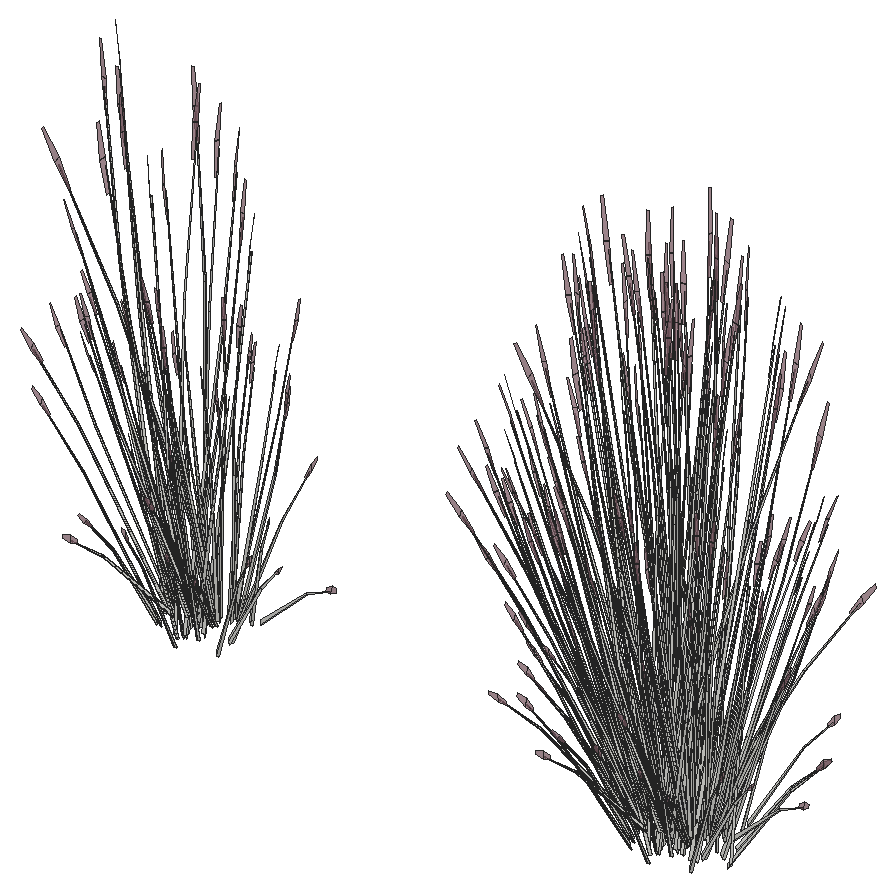
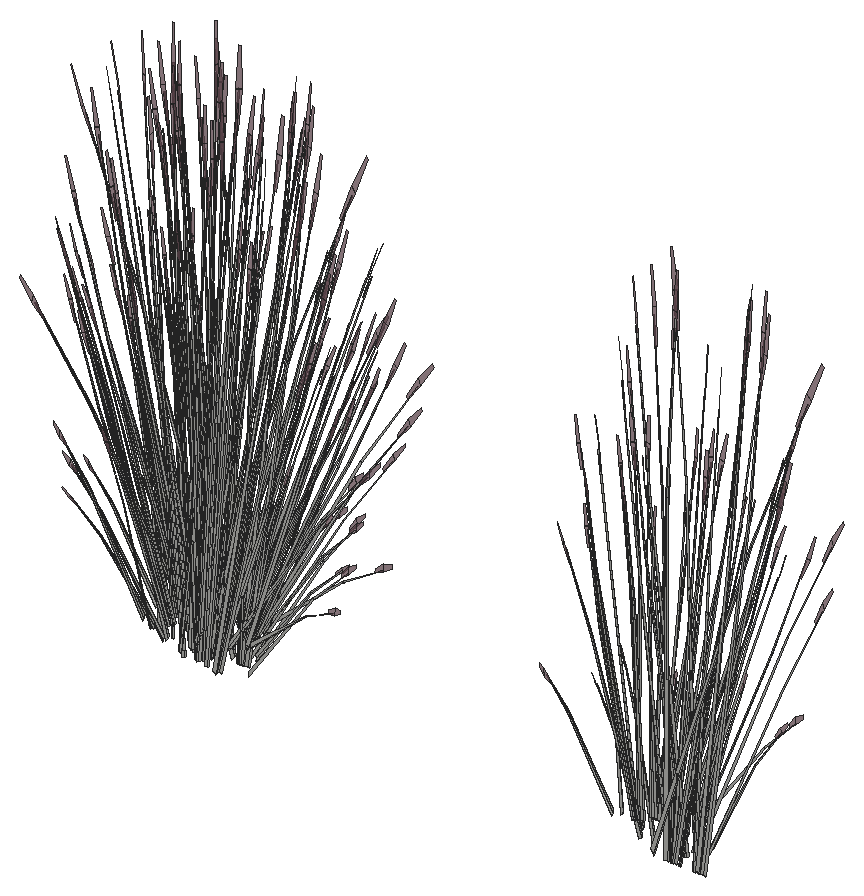
# SketchUp Ruby script. Lengths in inches.
U = 1.inch
M = Sketchup.active_model
def pt(a) = Geom::Point3d.new(a.map { |v| v * U })
def face(e, loops, mat)
  f = e.add_face(loops[0].map { |a| pt(a) })
  loops[1..].each { |l| e.add_face(l.map { |a| pt(a) }).erase! }
  f.material = f.back_material = mat if mat
  f
end
# faces: each face lists its corners as indices into pts; further lists are holes
def faces(e, pts, list, mat = nil) = list.each { |f| face(e, (f[0].is_a?(Array) ? f : [f]).map { |l| l.map { |i| pts[i] } }, mat) }
# xy, xz, yz: faces in a plane at the given z, y or x. An outline is a flat list of corners, or four numbers for a rectangle; further outlines are holes
def ring(l) = l.size == 4 ? [[l[0], l[1]], [l[2], l[1]], [l[2], l[3]], [l[0], l[3]]] : l.each_slice(2).to_a
def flat(e, list, mat, &to3) = list.each { |f| face(e, (f[0].is_a?(Array) ? f : [f]).map { |l| ring(l).map { |u, v| to3.(u, v) } }, mat) }
def xy(e, z, list, mat = nil) = flat(e, list, mat) { |x, y| [x, y, z] }
def xz(e, y, list, mat = nil) = flat(e, list, mat) { |x, z| [x, y, z] }
def yz(e, x, list, mat = nil) = flat(e, list, mat) { |y, z| [x, y, z] }
def lines(e, pts, list) = list.each { |a, b| e.add_line(pt(pts[a]), pt(pts[b])) }
# prism: a flat outline (further loops are holes) pulled along v
def prism(e, loops, v, mat = nil)
  f = face(e, loops, mat); d = Geom::Vector3d.new(v.map { |x| x * U })
  f.pushpull(f.normal.samedirection?(d) ? d.length : -d.length)
end
def box(e, o, s, mat = nil) = prism(e, [[o, [o[0] + s[0], o[1], o[2]], [o[0] + s[0], o[1] + s[1], o[2]], [o[0], o[1] + s[1], o[2]]]], [0, 0, s[2]], mat)
def at(x, y, z, deg = 0) = Geom::Transformation.translation(pt([x, y, z])) * Geom::Transformation.rotation(ORIGIN, Z_AXIS, deg.degrees)
def axes(o, x, y, z) = Geom::Transformation.new([*x, 0, *y, 0, *z, 0, *pt(o).to_a, 1])
def part(name) = M.definitions.add(name)
# library, detail: a bought-in or finely detailed component or shape, given as its bounding box
def library(name, o, s) = part(name).tap { |d| box(d.entities, o, s) }
def detail(e, o, s) = box(e.add_group.entities, o, s)
def put(e, d, t, mat = nil) = e.add_instance(d, t).tap { |i| i.material = mat if mat }
def group(e, t, mat = nil) = e.add_group.tap { |g| g.transformation = t; g.material = mat if mat }.entities
root = M.entities
M.materials.add("LightPink_Translucent").color = [144, 107, 117]
M.materials["LightPink_Translucent"].alpha = 0.75
c1 = part("blade")
p = [[2.15,0.21,22],[0,0.17,0],[0.09,0.45,0],[2.18,0.31,22],[2.29,0.31,22],[0.38,0.45,0],
  [2.48,0.24,33],[2.49,0.24,33],[2.48,0.22,33]]
faces(c1.entities,p,[[0,1,2,3],[4,5,2,3],[6,3,4,7],[8,0,3,6]])
c2 = part("seeds")
p = [[0.3,-0.1,1.38],[-0.01,-0.03,1.59],[-0.01,-0.03,0.03],[0.14,-0.07,-0.07],[0.29,-0.03,3],[0.15,0.01,3.11]]
faces(c2.entities,p,[[0,1,2,3],[1,0,4,5]],"LightPink_Translucent")
c3 = part("blade with seeds")
put(c3.entities,c1,at(0,0,0))
put(c3.entities,c2,axes([2.4,0.25,30.99],[1.5799,-0.05474,1.17369],[-0.12525,1.92788,0.29478],[-0.07173,-0.02425,1.56792]))
put(root,c3,axes([752.32,276.33,1.9375],[0.10505,0.10498,0.85688],[-0.48542,0.08838,0.06928],[-0.10971,-0.1648,0.36631]))
put(root,c3,axes([753.12,275.64,2.36],[-0.07029,-0.04584,0.87472],[-0.46908,0.02906,-0.13834],[-0.07486,-0.10965,0.07015]))
put(root,c3,axes([754.21,276.18,1.3],[-0.13063,0.06618,0.71501],[-0.39122,-0.11583,-0.15377],[0.07252,-0.14406,0.3057]))
put(root,c3,axes([753.61,276.41,2.49],[-0.21934,-0.26585,-0.35523],[0.45151,-0.14816,0.04287],[-0.05129,-0.12845,0.5025]))
put(root,c3,axes([752.18,276.05,1.3],[-0.02783,0.10696,0.71501],[-0.40683,0.08954,-0.15377],[-0.0951,-0.13825,0.3057]))
put(root,c3,axes([753.23,275.82,0.75],[-0.07708,0.01178,0.88171],[-0.42627,-0.1326,-0.1347],[0.00715,-0.1106,0.15018]))
put(root,c3,axes([754.52,276.67,2.49],[0.01196,-0.30243,-0.35523],[0.50354,0.02031,0.04287],[0.05314,-0.12813,0.5025]))
put(root,c3,axes([755.23,276.2,2.36],[-0.00444,-0.06507,0.87472],[-0.37468,-0.18807,-0.13834],[0.05793,-0.114,0.07015]))
put(root,c3,axes([753.65,276.18,2.26],[0.13855,-0.25143,-0.17707],[0.4042,0.07334,0.2286],[-0.03706,-0.10123,0.4374]))
put(root,c3,axes([753.96,276.52,1.9375],[-0.08557,0.11238,0.85688],[-0.35897,-0.23257,0.06928],[0.16194,-0.14495,0.36631]))
put(root,c3,axes([755.125,275.96,2.35],[-0.04667,0.02497,0.88692],[-0.45726,-0.08426,-0.08381],[-0.01655,-0.10898,0.15695]))
put(root,c3,axes([753.45,276.36,2.34],[-0.45175,-0.08196,-0.25549],[0.15485,-0.28101,-0.1979],[-0.04142,-0.11314,0.48886]))
put(root,c3,axes([753.73,275.65,1.38],[0.05895,0.19066,0.5743],[-0.32704,-0.1056,0.42196],[0.03519,-0.09762,0.12649]))
put(root,c3,axes([754.42,276.57,2.34],[-0.32898,-0.21969,-0.25549],[0.34753,-0.1924,-0.1979],[0.05006,-0.11162,0.48886]))
put(root,c3,axes([752.64,275.49,2.35],[-0.00857,0.03919,0.88692],[-0.42284,0.14223,-0.08381],[-0.12443,-0.0727,0.15695]))
put(root,c3,axes([752.54,276.18,2.55],[0.51193,-0.08404,0.26881],[0.08885,0.32966,0.22165],[-0.1204,-0.09716,0.55625]))
put(root,c3,axes([753.7,276.24,2.37],[0.45283,0.08548,0.24001],[-0.15485,0.28101,0.1979],[-0.02721,-0.11051,0.49665]))
put(root,c3,axes([753.83,276.34,2.52],[-0.44971,0.15222,-0.0608],[-0.221,-0.27017,-0.33747],[-0.05933,-0.11385,0.51278]))
put(root,c3,axes([754.77,276.6875,2.52],[-0.50507,-0.0162,-0.0608],[0.01381,-0.30672,-0.33747],[0.03508,-0.11813,0.51278]))
put(root,c3,axes([754.73,276.49,2.26],[0.31095,-0.17214,-0.17707],[0.29435,0.19656,0.2286],[0.04479,-0.09987,0.4374]))
put(root,c3,axes([752.04,275.88,1.38],[0.23972,0.1138,0.5743],[-0.34912,0.06841,0.42196],[-0.0747,-0.08746,0.12649]))
put(root,c3,axes([753.82,276.22,2.37],[0.33863,-0.11112,0.03215],[0.16575,0.20263,0.2531],[-0.0327,-0.08932,0.38595]))
put(root,c3,axes([752.62,276.49,2.49],[-0.39186,-0.15803,-0.35523],[0.27849,-0.27693,0.04287],[-0.14198,-0.09436,0.5025]))
put(root,c3,axes([752.49,276.28,2.26],[-0.07098,-0.26335,-0.17707],[0.40574,-0.06954,0.2286],[-0.10898,-0.07547,0.4374]))
put(root,c3,axes([752.66,276.25,2.37],[0.20887,-0.2077,0.03215],[0.29744,0.12092,0.2531],[-0.09616,-0.06659,0.38595]))
put(root,c3,axes([751.85,276.23,0.75],[-0.04451,0.04307,0.88171],[-0.44986,0.09286,-0.1347],[-0.10868,-0.08448,0.15018]))
put(root,c3,axes([752.6,277.41,1.05],[-0.18873,-0.33528,-0.34918],[0.54365,-0.12075,-0.09164],[-0.02086,-0.11353,0.77075]))
put(root,c3,axes([751.61,276.66,1.9375],[0.1707,0.05633,0.85688],[-0.35326,0.23632,0.06928],[-0.22018,-0.10661,0.36631]))
put(root,c3,axes([755.12,276.38,0.75],[-0.06878,-0.02576,0.88171],[-0.17668,-0.28776,-0.1347],[0.11919,-0.07809,0.15018]))
put(root,c3,axes([753.7,276.45,2.53],[-0.13855,0.25143,0.17707],[-0.4042,-0.07334,-0.2286],[-0.03706,-0.10123,0.4374]))
put(root,c3,axes([752.4375,276.49,2.34],[-0.45348,0.07772,-0.25549],[-0.07933,-0.29434,-0.1979],[-0.1218,-0.08435,0.48886]))
put(root,c3,axes([754.73,276.56,2.37],[0.32725,0.22308,0.24001],[-0.34753,0.1924,0.1979],[0.06036,-0.10466,0.49665]))
put(root,c3,axes([752.76,276.23,2.72],[-0.30671,0.31344,-0.0681],[-0.44417,-0.18058,-0.37797],[-0.1544,-0.08856,0.57432]))
put(root,c3,axes([754.85,276.58,2.37],[0.37765,0.01523,0.03215],[-0.01035,0.23004,0.2531],[0.03952,-0.08812,0.38595]))
put(root,c3,axes([754.57,276.73,2.53],[-0.31095,0.17214,0.17707],[-0.29435,-0.19656,-0.2286],[0.04479,-0.09987,0.4374]))
put(root,c3,axes([755.12,277.2,2.49],[0.24005,-0.25798,-0.35523],[0.42065,0.18334,0.04287],[0.14333,-0.09347,0.5025]))
put(root,c3,axes([752.52,276.45,1.1875],[-0.28732,-0.32763,0],[0.4807,-0.18271,-0.25804],[0.10948,-0.04161,0.81856]))
put(root,c3,axes([755.11,277.08,2.34],[-0.11806,-0.29854,-0.25549],[0.44709,-0.05222,-0.1979],[0.12812,-0.08019,0.48886]))
put(root,c3,axes([753.15,276.05,1.0625],[-0.31757,0.18757,-0.01946],[-0.29098,-0.20543,-0.08825],[-0.02049,-0.05821,0.29107]))
put(root,c3,axes([751.58,276.14,2.36],[-0.09888,-0.00231,0.87472],[-0.3148,0.23079,-0.13834],[-0.16797,-0.04716,0.07015]))
put(root,c3,axes([755.32,277.29,2.52],[-0.4251,-0.18028,-0.0608],[0.24491,-0.26108,-0.33747],[0.1201,-0.09075,0.51278]))
put(root,c3,axes([753.56,278.27,1.66],[0.39713,0.13184,0.7563],[-0.38905,0.28403,0.29908],[-0.17427,-0.16834,0.63403]))
put(root,c3,axes([752.73,276.49,2.53],[0.07098,0.26335,0.17707],[-0.40574,0.06954,-0.2286],[-0.10898,-0.07547,0.4374]))
put(root,c3,axes([751.48,277.36,1.01],[0,-0.32696,-0.24825],[0.51416,0,0],[0,-0.07447,0.78752]))
put(root,c3,axes([752.91,276.39,1.01],[0.4301,-0.16348,-0.24825],[0.25708,0.29314,0],[0.09796,-0.03723,0.78752]))
put(root,c3,axes([755.46,276.96,1.3],[-0.16417,-0.00968,0.71501],[-0.16819,-0.25979,-0.15377],[0.20169,-0.07349,0.3057]))
put(root,c3,axes([751.51,276.66,2.55],[0.37952,-0.24129,0.26881],[0.32731,0.25625,0.22165],[-0.17806,-0.04451,0.55625]))
put(root,c3,axes([756.36,277.21,2.35],[-0.06002,-0.00248,0.88692],[-0.24926,-0.26607,-0.08381],[0.1001,-0.08748,0.15695]))
put(root,c3,axes([724.19,278.45,1.9375],[0.10505,0.10498,0.85688],[-0.48542,0.08838,0.06928],[-0.10971,-0.1648,0.36631]))
put(root,c3,axes([753.42,277.06,1.03],[0.30954,-0.24575,-0.31177],[0.38452,0.22284,-0.08182],[0.12404,-0.0613,0.68817]))
put(root,c3,axes([755.65,276.48,1.38],[-0.15307,0.16644,0.5743],[-0.13157,-0.22361,0.42196],[0.12643,-0.05603,0.12649]))
put(root,c3,axes([725,277.75,2.36],[-0.07029,-0.04584,0.87472],[-0.46908,0.02906,-0.13834],[-0.07486,-0.10965,0.07015]))
put(root,c3,axes([726.08,278.3,1.3],[-0.13063,0.06618,0.71501],[-0.39122,-0.11583,-0.15377],[0.07252,-0.14406,0.3057]))
put(root,c3,axes([725.49,278.53,2.49],[-0.21934,-0.26585,-0.35523],[0.45151,-0.14816,0.04287],[-0.05129,-0.12845,0.5025]))
put(root,c3,axes([755.43,277.11,2.26],[0.40003,-0.04673,-0.17707],[0.10563,0.26712,0.2286],[0.11464,-0.07175,0.4374]))
put(root,c3,axes([751.68,276.66,2.37],[0.02314,-0.24862,0.03215],[0.34943,0.00682,0.2531],[-0.13385,-0.02602,0.38595]))
put(root,c3,axes([724.0625,278.17,1.3],[-0.02783,0.10696,0.71501],[-0.40683,0.08954,-0.15377],[-0.0951,-0.13825,0.3057]))
put(root,c3,axes([752.88,277.5,1.11],[0.22297,-0.29461,-0.2237],[0.4633,0.14179,0.10766],[0,-0.06791,0.71822]))
put(root,c3,axes([751.55,276.74,2.26],[-0.26148,-0.20471,-0.17707],[0.29857,-0.19378,0.2286],[-0.1517,-0.02948,0.4374]))
put(root,c3,axes([753.09,277.35,1.33],[-0.05355,-0.37308,-0.14548],[0.55775,-0.02256,-0.25001],[0.09822,-0.04969,0.79854]))
put(root,c3,axes([725.11,277.9375,0.75],[-0.07708,0.01178,0.88171],[-0.42627,-0.1326,-0.1347],[0.00715,-0.1106,0.15018]))
put(root,c3,axes([751.7,277.37,1.01],[0.32079,-0.20399,-0.15489],[0.32079,0.20399,0.15489],[0,-0.06571,0.69487]))
put(root,c3,axes([751.57,276.39,1.0625],[-0.13257,0.26698,-0.01946],[-0.40802,-0.08212,-0.08825],[-0.06195,-0.04367,0.29107]))
put(root,c3,axes([755.11,277.26,2.53],[-0.40003,0.04673,0.17707],[-0.10563,-0.26712,-0.2286],[0.11464,-0.07175,0.4374]))
put(root,c3,axes([752.83,277.74,1.33],[-0.51755,-0.15601,-0.14548],[0.2492,-0.32927,-0.25001],[-0.01626,-0.08084,0.79854]))
put(root,c3,axes([751.36,277.61,1.1875],[-0.57465,0,0],[0,-0.36542,-0.25804],[0,-0.08323,0.81856]))
put(root,c3,axes([726.4,278.79,2.49],[0.01196,-0.30243,-0.35523],[0.50354,0.02031,0.04287],[0.05314,-0.12813,0.5025]))
put(root,c3,axes([751.45,276.96,1.3],[0.08973,0.09103,0.71501],[-0.20675,0.24743,-0.15377],[-0.2123,-0.05914,0.3057]))
put(root,c3,axes([753.01,276.52,1.01],[0.42874,0.0809,-0.15489],[-0.10795,0.28489,0.15489],[0.08643,-0.03285,0.69487]))
put(root,c3,axes([727.1,278.31,2.36],[-0.00444,-0.06507,0.87472],[-0.37468,-0.18807,-0.13834],[0.05793,-0.114,0.07015]))
put(root,c3,axes([725.53,278.3,2.26],[0.13855,-0.25143,-0.17707],[0.4042,0.07334,0.2286],[-0.03706,-0.10123,0.4374]))
put(root,c3,axes([725.83,278.63,1.9375],[-0.08557,0.11238,0.85688],[-0.35897,-0.23257,0.06928],[0.16194,-0.14495,0.36631]))
put(root,c3,axes([727,278.08,2.35],[-0.04667,0.02497,0.88692],[-0.45726,-0.08426,-0.08381],[-0.01655,-0.10898,0.15695]))
put(root,c3,axes([751.82,276.875,2.49],[-0.45939,-0.00787,-0.35523],[0.03085,-0.3315,0.04287],[-0.19462,-0.03498,0.5025]))
put(root,c3,axes([725.32,278.47,2.34],[-0.45175,-0.08196,-0.25549],[0.15485,-0.28101,-0.1979],[-0.04142,-0.11314,0.48886]))
put(root,c3,axes([725.6,277.77,1.38],[0.05895,0.19066,0.5743],[-0.32704,-0.1056,0.42196],[0.03519,-0.09762,0.12649]))
put(root,c3,axes([726.3,278.6875,2.34],[-0.32898,-0.21969,-0.25549],[0.34753,-0.1924,-0.1979],[0.05006,-0.11162,0.48886]))
put(root,c3,axes([755.47,277.22,2.37],[0.31549,0.13751,0.03215],[-0.18368,0.19581,0.2531],[0.10115,-0.06331,0.38595]))
put(root,c3,axes([755.38,277.16,2.37],[0.11397,0.30091,0.24001],[-0.44709,0.05222,0.1979],[0.13177,-0.07077,0.49665]))
put(root,c3,axes([756.59,277.53,2.36],[0.06377,-0.0498,0.87472],[-0.08162,-0.30549,-0.13834],[0.16001,-0.05792,0.07015]))
put(root,c3,axes([751.8,277.51,1.17],[-0.42746,0.27488,0.15378],[-0.42772,-0.27199,-0.18246],[-0.01493,-0.07806,0.82443]))
put(root,c3,axes([751.2,276.34,2.35],[0.03407,0.03263,0.88692],[-0.16424,0.29331,-0.08381],[-0.16634,0.00212,0.15695]))
put(root,c3,axes([724.42,278.3,2.55],[0.51193,-0.08404,0.26881],[0.08885,0.32966,0.22165],[-0.1204,-0.09716,0.55625]))
put(root,c3,axes([725.58,278.36,2.37],[0.45283,0.08548,0.24001],[-0.15485,0.28101,0.1979],[-0.02721,-0.11051,0.49665]))
put(root,c3,axes([725.71,278.46,2.52],[-0.44971,0.15222,-0.0608],[-0.221,-0.27017,-0.33747],[-0.05933,-0.11385,0.51278]))
put(root,c3,axes([753.16,277.64,1.22],[0.5178,0.15847,0.12032],[-0.2492,0.32927,0.25001],[0,-0.0759,0.80271]))
put(root,c3,axes([752.96,278.09,1.22],[0.1218,-0.38743,-0.11714],[0.57753,0.06753,0.25635],[-0.10091,-0.0535,0.7822]))
put(root,c3,axes([726.64,278.8,2.52],[-0.50507,-0.0162,-0.0608],[0.01381,-0.30672,-0.33747],[0.03508,-0.11813,0.51278]))
put(root,c3,axes([726.61,278.61,2.26],[0.31095,-0.17214,-0.17707],[0.29435,0.19656,0.2286],[0.04479,-0.09987,0.4374]))
put(root,c3,axes([723.92,278,1.38],[0.23972,0.1138,0.5743],[-0.34912,0.06841,0.42196],[-0.0747,-0.08746,0.12649]))
put(root,c3,axes([725.7,278.34,2.37],[0.33863,-0.11112,0.03215],[0.16575,0.20263,0.2531],[-0.0327,-0.08932,0.38595]))
put(root,c3,axes([751.67,276.94,2.34],[-0.3337,0.21658,-0.25549],[-0.29224,-0.22879,-0.1979],[-0.16955,-0.03295,0.48886]))
put(root,c3,axes([724.36,278.39,2.26],[-0.07098,-0.26335,-0.17707],[0.40574,-0.06954,0.2286],[-0.10898,-0.07547,0.4374]))
put(root,c3,axes([751.92,276.85,2.53],[0.26148,0.20471,0.17707],[-0.29857,0.19378,-0.2286],[-0.1517,-0.02948,0.4374]))
put(root,c3,axes([750.92,277.23,1.38],[0.2934,-0.0234,0.5743],[-0.18611,0.20614,0.42196],[-0.14499,-0.03092,0.12649]))
put(root,c3,axes([752.99,277.42,1.36],[-0.49904,0.02018,0.2237],[-0.04513,-0.33504,-0.10766],[0.08934,-0.03396,0.71822]))
put(root,c3,axes([751.85,276.72,2.52],[-0.02461,0.33251,-0.0608],[-0.4659,-0.00909,-0.33747],[-0.17944,-0.0231,0.51278]))
put(root,c3,axes([751.7,277.67,1.24],[0,0.32696,0.24825],[-0.51416,0,0],[0,-0.07447,0.78752]))
put(root,c3,axes([755.33,277.99,2.52],[-0.23123,-0.29606,-0.0608],[0.41039,-0.14549,-0.33747],[0.17294,-0.03906,0.51278]))
put(root,c3,axes([755.3125,277.74,2.34],[0.1245,-0.29741,-0.25549],[0.42685,0.10194,-0.1979],[0.17186,-0.02727,0.48886]))
put(root,c3,axes([754.64,276.53,1.1875],[0.28732,-0.32763,0],[0.4807,0.18271,-0.25804],[0.10948,0.04161,0.81856]))
put(root,c3,axes([751.25,277.17,1.9375],[0.19062,-0.00741,0.85688],[-0.12645,0.32094,0.06928],[-0.27165,-0.01985,0.36631]))
put(root,c3,axes([752.92,277.93,1.11],[-0.27607,-0.27443,-0.2237],[0.41817,-0.19325,0.10766],[-0.08934,-0.03396,0.71822]))
put(root,c3,axes([752.97,277.54,1.18],[0.1998,0.3656,0.22877],[-0.5709,0.12713,0.08977],[0.00698,-0.06718,0.79428]))
put(root,c3,axes([724.54,278.37,2.37],[0.20887,-0.2077,0.03215],[0.29744,0.12092,0.2531],[-0.09616,-0.06659,0.38595]))
put(root,c3,axes([755.77,277.82,0.99],[-0.29599,0.03924,0.70792],[-0.04711,-0.31232,0.04052],[0.20731,-0.04727,0.40283]))
put(root,c3,axes([756.31,277.55,1.13],[-0.28491,-0.20907,-0.03244],[0.31204,-0.19157,-0.14708],[0.08842,-0.01349,0.48512]))
put(root,c3,axes([724.47,279.53,1.05],[-0.18873,-0.33528,-0.34918],[0.54365,-0.12075,-0.09164],[-0.02086,-0.11353,0.77075]))
put(root,c3,axes([727,278.5,0.75],[-0.06878,-0.02576,0.88171],[-0.17668,-0.28776,-0.1347],[0.11919,-0.07809,0.15018]))
put(root,c3,axes([752.875,277.83,1.36],[-0.22297,0.29461,0.2237],[-0.4633,-0.14179,-0.10766],[0,-0.06791,0.71822]))
put(root,c3,axes([753.69,277.57,1.1],[0,-0.37831,0],[0.57465,0,0],[0,0,0.89728]))
put(root,c3,axes([754.39,276.7,1.24],[-0.4301,-0.16348,0.24825],[0.25708,-0.29314,0],[0.09796,0.03723,0.78752]))
put(root,c3,axes([725.57,278.57,2.53],[-0.13855,0.25143,0.17707],[-0.4042,-0.07334,-0.2286],[-0.03706,-0.10123,0.4374]))
put(root,c3,axes([755.23,277.85,2.49],[0.40382,-0.1444,-0.35523],[0.22505,0.29724,0.04287],[0.19512,-0.03377,0.5025]))
put(root,c3,axes([726.61,278.67,2.37],[0.32725,0.22308,0.24001],[-0.34753,0.1924,0.1979],[0.06036,-0.10466,0.49665]))
put(root,c3,axes([752.67,278.03,1.03],[-0.47805,-0.0536,-0.31177],[0.10088,-0.33065,-0.08182],[-0.14266,-0.04007,0.68817]))
put(root,c3,axes([726.73,278.69,2.37],[0.37765,0.01523,0.03215],[-0.01035,0.23004,0.2531],[0.03952,-0.08812,0.38595]))
put(root,c3,axes([753.42,277.33,1.18],[-0.38104,0.29672,0.22877],[-0.45269,-0.26192,0.08977],[0.09186,-0.02961,0.79428]))
put(root,c3,axes([753.84,277.87,1.15],[-0.42746,-0.28142,-0.03066],[0.42772,-0.28159,0],[-0.01493,-0.00983,0.87786]))
put(root,c3,axes([726.45,278.85,2.53],[-0.31095,0.17214,0.17707],[-0.29435,-0.19656,-0.2286],[0.04479,-0.09987,0.4374]))
put(root,c3,axes([752.76,276.85,1.24],[-0.13276,0.32494,0.08821],[-0.4858,-0.09195,0.17543],[0.08392,-0.00158,0.80203]))
put(root,c3,axes([755.17,277.9,2.53],[-0.38192,-0.09121,0.17707],[0.11139,-0.2661,-0.2286],[0.15377,-0.0244,0.4374]))
put(root,c3,axes([726.99,279.3125,2.49],[0.24005,-0.25798,-0.35523],[0.42065,0.18334,0.04287],[0.14333,-0.09347,0.5025]))
put(root,c3,axes([724.4,278.5625,1.1875],[-0.28732,-0.32763,0],[0.4807,-0.18271,-0.25804],[0.10948,-0.04161,0.81856]))
put(root,c3,axes([726.98,279.19,2.34],[-0.11806,-0.29854,-0.25549],[0.44709,-0.05222,-0.1979],[0.12812,-0.08019,0.48886]))
put(root,c3,axes([751.17,277.42,2.37],[0.12984,-0.29812,0.24001],[0.42685,0.10194,0.1979],[-0.16786,0.01792,0.49665]))
put(root,c3,axes([752.56,277.11,0.8],[-0.45234,0.1309,0.64464],[-0.14398,-0.37559,0.25048],[0.27777,0.00625,0.73321]))
put(root,c3,axes([753.77,277.21,1.31],[0.08866,-0.29179,0.0724],[0.43315,0.05065,-0.20674],[0.07883,0.02996,0.63372]))
put(root,c3,axes([725.03,278.17,1.0625],[-0.31757,0.18757,-0.01946],[-0.29098,-0.20543,-0.08825],[-0.02049,-0.05821,0.29107]))
put(root,c3,axes([751.14,277.34,2.37],[-0.16879,-0.22293,0.03215],[0.30779,-0.10912,0.2531],[-0.13568,0.02153,0.38595]))
put(root,c3,axes([753.02,277.9,1.18],[0.58084,0.06889,0.22877],[-0.11821,0.38906,0.08977],[-0.08488,-0.03757,0.79428]))
put(root,c3,axes([756.09,277.62,0.75],[-0.02402,-0.04964,0.88171],[0.16658,-0.29036,-0.1347],[0.16804,-0.00418,0.15018]))
put(root,c3,axes([727.19,279.41,2.52],[-0.4251,-0.18028,-0.0608],[0.24491,-0.26108,-0.33747],[0.1201,-0.09075,0.51278]))
put(root,c3,axes([751.13,277.57,0.75],[0.01165,0.05153,0.88171],[-0.23495,0.26909,-0.1347],[-0.16689,-0.01356,0.15018]))
put(root,c3,axes([753.59,277.28,1.36],[-0.27607,-0.27443,0.2237],[0.41817,-0.19325,-0.10766],[0.08934,0.03396,0.71822]))
put(root,c3,axes([752.16,278.54,1.01],[-0.10795,-0.28489,-0.15489],[0.42874,-0.0809,0.15489],[-0.08643,-0.03285,0.69487]))
put(root,c3,axes([725.4375,280.39,1.66],[0.39713,0.13184,0.7563],[-0.38905,0.28403,0.29908],[-0.17427,-0.16834,0.63403]))
put(root,c3,axes([752.71,278.52,1.24],[0.49383,-0.08678,0.08821],[0.12194,0.32295,0.17543],[-0.04404,-0.04705,0.80203]))
put(root,c3,axes([753.73,277.3,1.33],[0.46399,-0.21707,-0.14548],[0.30855,0.30672,-0.25001],[0.11448,0.03115,0.79854]))
put(root,c3,axes([755.57,277.875,2.26],[0.38192,0.09121,-0.17707],[-0.11139,0.2661,0.2286],[0.15377,-0.0244,0.4374]))
put(root,c3,axes([724.6,278.61,2.53],[0.07098,0.26335,0.17707],[-0.40574,0.06954,-0.2286],[-0.10898,-0.07547,0.4374]))
put(root,c3,axes([723.36,279.48,1.01],[0,-0.32696,-0.24825],[0.51416,0,0],[0,-0.07447,0.78752]))
put(root,c3,axes([724.79,278.51,1.01],[0.4301,-0.16348,-0.24825],[0.25708,0.29314,0],[0.09796,-0.03723,0.78752]))
put(root,c3,axes([727.34,279.08,1.3],[-0.16417,-0.00968,0.71501],[-0.16819,-0.25979,-0.15377],[0.20169,-0.07349,0.3057]))
put(root,c3,axes([728.24,279.33,2.35],[-0.06002,-0.00248,0.88692],[-0.24926,-0.26607,-0.08381],[0.1001,-0.08748,0.15695]))
put(root,c3,axes([752.04,278.66,1.01],[-0.4301,-0.16348,-0.24825],[0.25708,-0.29314,0],[-0.09796,-0.03723,0.78752]))
put(root,c3,axes([754.9,276.72,1.01],[0.4301,0.16348,-0.24825],[-0.25708,0.29314,0],[0.09796,0.03723,0.78752]))
put(root,c3,axes([751.09,277.45,2.26],[-0.38192,-0.09121,-0.17707],[0.11139,-0.2661,0.2286],[-0.15377,0.0244,0.4374]))
put(root,c3,axes([754.08,277.66,1.1],[0.51416,0,0],[0,0.33849,0],[0,0,0.89203]))
put(root,c3,axes([725.3,279.18,1.03],[0.30954,-0.24575,-0.31177],[0.38452,0.22284,-0.08182],[0.12404,-0.0613,0.68817]))
put(root,c3,axes([753.21,278.08,1.33],[-0.46399,0.21707,-0.14548],[-0.30855,-0.30672,-0.25001],[-0.11448,-0.03115,0.79854]))
put(root,c3,axes([754.23,276.86,1.24],[-0.49383,0.08678,0.08821],[-0.12194,-0.32295,0.17543],[0.04404,0.04705,0.80203]))
put(root,c3,axes([727.53,278.6,1.38],[-0.15307,0.16644,0.5743],[-0.13157,-0.22361,0.42196],[0.12643,-0.05603,0.12649]))
put(root,c3,axes([754.53,277.54,1.9375],[-0.19062,0.00741,0.85688],[0.12645,-0.32094,0.06928],[0.27165,0.01985,0.36631]))
put(root,c3,axes([754.78,276.85,1.01],[0.10795,0.28489,-0.15489],[-0.42874,0.0809,0.15489],[0.08643,0.03285,0.69487]))
put(root,c3,axes([727.3125,279.22,2.26],[0.40003,-0.04673,-0.17707],[0.10563,0.26712,0.2286],[0.11464,-0.07175,0.4374]))
put(root,c3,axes([755.52,277.99,2.37],[0.16879,0.22293,0.03215],[-0.30779,0.10912,0.2531],[0.13568,-0.02153,0.38595]))
put(root,c3,axes([753.92,277.49,1.19],[-0.58084,-0.06889,0.24599],[0.11821,-0.38906,0.09653],[0.08488,0.03757,0.85407]))
put(root,c3,axes([724.76,279.61,1.11],[0.22297,-0.29461,-0.2237],[0.4633,0.14179,0.10766],[0,-0.06791,0.71822]))
put(root,c3,axes([755.49,277.91,2.37],[-0.12984,0.29812,0.24001],[-0.42685,-0.10194,0.1979],[0.16786,-0.01792,0.49665]))
put(root,c3,axes([753.45,278.45,1.1],[-0.14994,-0.28188,0],[0.42817,-0.09871,0],[0,0,0.77185]))
put(root,c3,axes([724.96,279.47,1.33],[-0.05355,-0.37308,-0.14548],[0.55775,-0.02256,-0.25001],[0.09822,-0.04969,0.79854]))
put(root,c3,axes([723.58,279.49,1.01],[0.32079,-0.20399,-0.15489],[0.32079,0.20399,0.15489],[0,-0.06571,0.69487]))
put(root,c3,axes([753.17,278.18,1.31],[-0.08866,0.29179,0.0724],[-0.43315,-0.05065,-0.20674],[-0.07883,-0.02996,0.63372]))
put(root,c3,axes([751.49,277.42,2.53],[0.38192,0.09121,0.17707],[-0.11139,0.2661,-0.2286],[-0.15377,0.0244,0.4374]))
put(root,c3,axes([754.02,278.41,1.09],[0.48247,-0.11094,-0.09599],[0.16954,0.31956,0.00004],[0.05326,-0.01226,0.86949]))
put(root,c3,axes([726.99,279.38,2.53],[-0.40003,0.04673,0.17707],[-0.10563,-0.26712,-0.2286],[0.11464,-0.07175,0.4374]))
put(root,c3,axes([724.71,279.86,1.33],[-0.51755,-0.15601,-0.14548],[0.2492,-0.32927,-0.25001],[-0.01626,-0.08084,0.79854]))
put(root,c3,axes([754.18,278.54,1.24],[0.13276,-0.32494,0.08821],[0.4858,0.09195,0.17543],[-0.08392,0.00158,0.80203]))
put(root,c3,axes([723.23,279.73,1.1875],[-0.57465,0,0],[0,-0.36542,-0.25804],[0,-0.08323,0.81856]))
put(root,c3,axes([754.07,277.8,1.11],[0.32079,0.21119,0],[-0.32079,0.21119,0],[0,0,0.84633]))
put(root,c3,axes([752.25,277.41,1.67],[0.13063,-0.0473,0.88532],[0.04505,0.33024,0.06928],[-0.28294,0.04382,0.31642]))
put(root,c3,axes([754.94,277.71,1.24],[-0.36107,-0.23816,0.08821],[0.36387,-0.231,0.17543],[-0.03988,0.04864,0.80203]))
put(root,c3,axes([724.89,278.64,1.01],[0.42874,0.0809,-0.15489],[-0.10795,0.28489,0.15489],[0.08643,-0.03285,0.69487]))
put(root,c3,axes([754.27,277.35,1.03],[0.47805,0.0536,-0.31177],[-0.10088,0.33065,-0.08182],[0.14266,0.04007,0.68817]))
put(root,c3,axes([756.38,277.93,1.38],[-0.28394,0.05398,0.5743],[0.13365,-0.22308,0.42196],[0.15063,0.01526,0.12649]))
put(root,c3,axes([753.35,278.57,1.1],[-0.4633,-0.14679,0],[0.22297,-0.30501,0],[0,0,0.81353]))
put(root,c3,axes([753.73,278.18,1.23],[-0.44875,-0.26316,-0.12596],[0.3776,-0.2955,0.27565],[-0.12084,0.03078,0.84108]))
put(root,c3,axes([752.55,278.6875,1.24],[0.4301,0.16348,0.24825],[-0.25708,0.29314,0],[-0.09796,-0.03723,0.78752]))
put(root,c3,axes([754.07,277.56,1.36],[0.22297,-0.29461,0.2237],[0.4633,0.14179,-0.10766],[0,0.06791,0.71822]))
put(root,c3,axes([756.25,278.87,2.35],[-0.04155,-0.02862,0.88692],[0.0909,-0.30682,-0.08381],[0.16368,-0.0196,0.15695]))
put(root,c3,axes([727.35,279.34,2.37],[0.31549,0.13751,0.03215],[-0.18368,0.19581,0.2531],[0.10115,-0.06331,0.38595]))
put(root,c3,axes([727.26,279.28,2.37],[0.11397,0.30091,0.24001],[-0.44709,0.05222,0.1979],[0.13177,-0.07077,0.49665]))
put(root,c3,axes([728.47,279.65,2.36],[0.06377,-0.0498,0.87472],[-0.08162,-0.30549,-0.13834],[0.16001,-0.05792,0.07015]))
put(root,c3,axes([750.84,277.63,2.36],[-0.07505,0.04245,0.87472],[0.00638,0.31015,-0.13834],[-0.17202,0.04033,0.07015]))
put(root,c3,axes([753.98,277.72,1.15],[0,0.37813,-0.02818],[-0.57465,0,0],[0,0.01188,0.89684]))
put(root,c3,axes([751.35,277.59,2.34],[-0.1245,0.29741,-0.25549],[-0.42685,-0.10194,-0.1979],[-0.17186,0.02727,0.48886]))
put(root,c3,axes([751.33,277.33,2.52],[0.23123,0.29606,-0.0608],[-0.41039,0.14549,-0.33747],[-0.17294,0.03906,0.51278]))
put(root,c3,axes([754.02,277.46,1.11],[0.27607,0.27443,-0.2237],[-0.41817,0.19325,0.10766],[0.08934,0.03396,0.71822]))
put(root,c3,axes([755.89,278.62,1.96],[-0.08796,-0.27485,-0.01746],[0.41573,-0.06319,-0.07916],[0.08682,0.01742,0.26109]))
put(root,c3,axes([752.3,278.86,1.1875],[-0.28732,0.32763,0],[-0.4807,-0.18271,-0.25804],[-0.10948,-0.04161,0.81856]))
put(root,c3,axes([754.8125,278.61,2.52],[0.02461,-0.33251,-0.0608],[0.4659,0.00909,-0.33747],[0.17944,0.0231,0.51278]))
put(root,c3,axes([723.68,279.63,1.17],[-0.42746,0.27488,0.15378],[-0.42772,-0.27199,-0.18246],[-0.01493,-0.07806,0.82443]))
put(root,c3,axes([755.24,277.72,1.24],[0,-0.32696,0.24825],[0.51416,0,0],[0,0.07447,0.78752]))
put(root,c3,axes([753.95,277.96,1.36],[0.49904,-0.02018,0.2237],[0.04513,0.33504,-0.10766],[-0.08934,0.03396,0.71822]))
put(root,c3,axes([754.26,277.62,1.31],[0.42817,-0.09535,0.0724],[0.14994,0.27228,-0.20674],[0,0.05992,0.63372]))
put(root,c3,axes([754.74,278.48,2.53],[-0.26148,-0.20471,0.17707],[0.29857,-0.19378,-0.2286],[0.1517,0.02948,0.4374]))
put(root,c3,axes([725.04,279.76,1.22],[0.5178,0.15847,0.12032],[-0.2492,0.32927,0.25001],[0,-0.0759,0.80271]))
